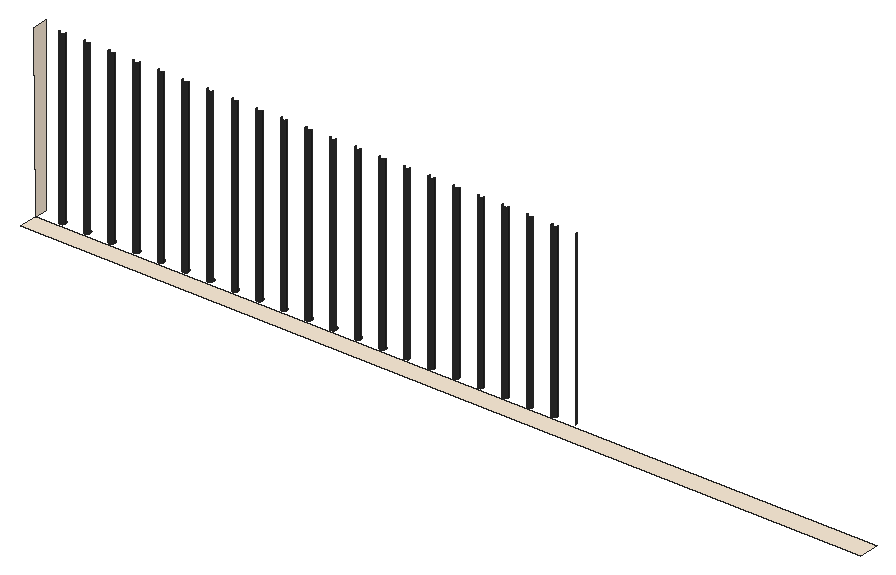
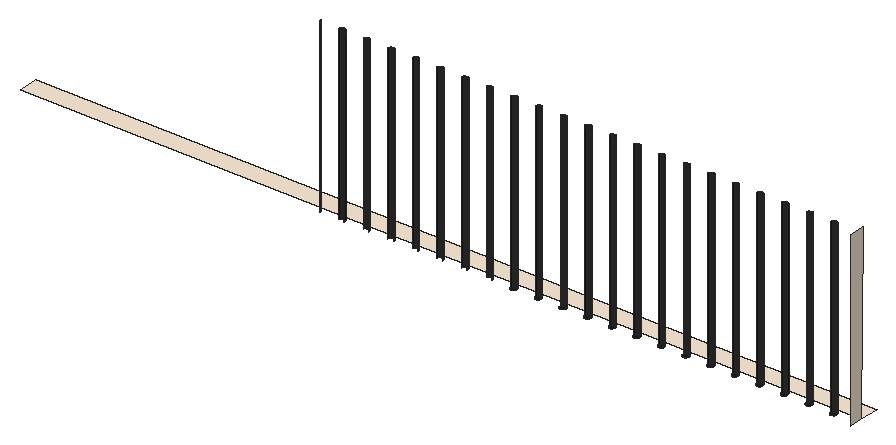
# SketchUp Ruby script. Lengths in inches.
U = 1.inch
M = Sketchup.active_model
def pt(a) = Geom::Point3d.new(a.map { |v| v * U })
def face(e, loops, mat)
  f = e.add_face(loops[0].map { |a| pt(a) })
  loops[1..].each { |l| e.add_face(l.map { |a| pt(a) }).erase! }
  f.material = f.back_material = mat if mat
  f
end
# faces: each face lists its corners as indices into pts; further lists are holes
def faces(e, pts, list, mat = nil) = list.each { |f| face(e, (f[0].is_a?(Array) ? f : [f]).map { |l| l.map { |i| pts[i] } }, mat) }
# xy, xz, yz: faces in a plane at the given z, y or x. An outline is a flat list of corners, or four numbers for a rectangle; further outlines are holes
def ring(l) = l.size == 4 ? [[l[0], l[1]], [l[2], l[1]], [l[2], l[3]], [l[0], l[3]]] : l.each_slice(2).to_a
def flat(e, list, mat, &to3) = list.each { |f| face(e, (f[0].is_a?(Array) ? f : [f]).map { |l| ring(l).map { |u, v| to3.(u, v) } }, mat) }
def xy(e, z, list, mat = nil) = flat(e, list, mat) { |x, y| [x, y, z] }
def xz(e, y, list, mat = nil) = flat(e, list, mat) { |x, z| [x, y, z] }
def yz(e, x, list, mat = nil) = flat(e, list, mat) { |y, z| [x, y, z] }
def lines(e, pts, list) = list.each { |a, b| e.add_line(pt(pts[a]), pt(pts[b])) }
# prism: a flat outline (further loops are holes) pulled along v
def prism(e, loops, v, mat = nil)
  f = face(e, loops, mat); d = Geom::Vector3d.new(v.map { |x| x * U })
  f.pushpull(f.normal.samedirection?(d) ? d.length : -d.length)
end
def box(e, o, s, mat = nil) = prism(e, [[o, [o[0] + s[0], o[1], o[2]], [o[0] + s[0], o[1] + s[1], o[2]], [o[0], o[1] + s[1], o[2]]]], [0, 0, s[2]], mat)
def at(x, y, z, deg = 0) = Geom::Transformation.translation(pt([x, y, z])) * Geom::Transformation.rotation(ORIGIN, Z_AXIS, deg.degrees)
def axes(o, x, y, z) = Geom::Transformation.new([*x, 0, *y, 0, *z, 0, *pt(o).to_a, 1])
def part(name) = M.definitions.add(name)
# library, detail: a bought-in or finely detailed component or shape, given as its bounding box
def library(name, o, s) = part(name).tap { |d| box(d.entities, o, s) }
def detail(e, o, s) = box(e.add_group.entities, o, s)
def put(e, d, t, mat = nil) = e.add_instance(d, t).tap { |i| i.material = mat if mat }
def group(e, t, mat = nil) = e.add_group.tap { |g| g.transformation = t; g.material = mat if mat }.entities
root = M.entities
M.materials.add("[0028_AntiqueWhite]").color = [250, 235, 215]
M.materials.add("[Color M08]").color = [30, 30, 30]
xy(root,177,[[50.75,190.5,206.5625,194.125]],"[0028_AntiqueWhite]")
xy(root,177,[[54.79,194.68,54.65,194.71,54.52,194.79,54.42,194.89,54.35,195.02,54.31,195.16,54.31,195.31,54.34,195.45,54.42,195.58,54.52,195.68,54.65,195.75,54.79,195.79,54.9375,195.79,55.08,195.75,55.21,195.68,55.31,195.58,55.38,195.45,55.42,195.31,55.42,195.16,55.38,195.02,55.3125,194.89,55.21,194.79,55.08,194.72,54.9375,194.68],[59.35,194.68,59.21,194.71,59.09,194.79,58.98,194.89,58.91,195.02,58.87,195.16,58.87,195.31,58.91,195.45,58.98,195.58,59.08,195.68,59.21,195.75,59.35,195.79,59.5,195.79,59.64,195.75,59.77,195.68,59.87,195.58,59.95,195.45,59.98,195.31,59.99,195.16,59.95,195.02,59.875,194.89,59.77,194.79,59.64,194.72,59.5,194.68],[63.92,194.68,63.78,194.71,63.65,194.79,63.54,194.89,63.47,195.02,63.43,195.16,63.43,195.31,63.47,195.45,63.54,195.58,63.65,195.68,63.77,195.75,63.92,195.79,64.0625,195.79,64.2,195.75,64.33,195.68,64.44,195.58,64.51,195.45,64.55,195.31,64.55,195.16,64.51,195.02,64.4375,194.89,64.33,194.79,64.21,194.72,64.0625,194.68],[68.48,194.68,68.34,194.71,68.21,194.79,68.11,194.89,68.03,195.02,67.99,195.16,67.99,195.31,68.03,195.45,68.11,195.58,68.21,195.68,68.34,195.75,68.48,195.79,68.625,195.79,68.77,195.75,68.89,195.68,69,195.58,69.07,195.45,69.11,195.31,69.11,195.16,69.07,195.02,69,194.89,68.9,194.79,68.77,194.72,68.625,194.68],[73.04,194.68,72.9,194.71,72.77,194.79,72.67,194.89,72.6,195.02,72.56,195.16,72.56,195.31,72.59,195.45,72.67,195.58,72.77,195.68,72.9,195.75,73.04,195.79,73.1875,195.79,73.33,195.75,73.46,195.68,73.56,195.58,73.63,195.45,73.67,195.31,73.67,195.16,73.63,195.02,73.5625,194.89,73.46,194.79,73.33,194.72,73.1875,194.68],
  [77.6,194.68,77.46,194.71,77.34,194.79,77.23,194.89,77.16,195.02,77.12,195.16,77.12,195.31,77.16,195.45,77.23,195.58,77.33,195.68,77.46,195.75,77.6,195.79,77.75,195.79,77.89,195.75,78.02,195.68,78.12,195.58,78.2,195.45,78.23,195.31,78.24,195.16,78.2,195.02,78.125,194.89,78.02,194.79,77.89,194.72,77.75,194.68],[82.17,194.68,82.03,194.71,81.9,194.79,81.79,194.89,81.72,195.02,81.68,195.16,81.68,195.31,81.72,195.45,81.79,195.58,81.9,195.68,82.02,195.75,82.17,195.79,82.3125,195.79,82.45,195.75,82.58,195.68,82.69,195.58,82.76,195.45,82.8,195.31,82.8,195.16,82.76,195.02,82.6875,194.89,82.58,194.79,82.46,194.72,82.3125,194.68],[86.73,194.68,86.59,194.71,86.46,194.79,86.36,194.89,86.28,195.02,86.24,195.16,86.24,195.31,86.28,195.45,86.36,195.58,86.46,195.68,86.59,195.75,86.73,195.79,86.875,195.79,87.02,195.75,87.14,195.68,87.25,195.58,87.32,195.45,87.36,195.31,87.36,195.16,87.32,195.02,87.25,194.89,87.15,194.79,87.02,194.72,86.875,194.68],[91.29,194.68,91.15,194.71,91.02,194.79,90.92,194.89,90.85,195.02,90.81,195.16,90.81,195.31,90.84,195.45,90.92,195.58,91.02,195.68,91.15,195.75,91.29,195.79,91.4375,195.79,91.58,195.75,91.71,195.68,91.81,195.58,91.88,195.45,91.92,195.31,91.92,195.16,91.88,195.02,91.8125,194.89,91.71,194.79,91.58,194.72,91.4375,194.68],[95.85,194.68,95.71,194.71,95.59,194.79,95.48,194.89,95.41,195.02,95.37,195.16,95.37,195.31,95.41,195.45,95.48,195.58,95.58,195.68,95.71,195.75,95.85,195.79,96,195.79,96.14,195.75,96.27,195.68,96.37,195.58,96.45,195.45,96.48,195.31,96.49,195.16,96.45,195.02,96.375,194.89,96.27,194.79,96.14,194.72,96,194.68],
  [100.42,194.68,100.28,194.71,100.15,194.79,100.04,194.89,99.97,195.02,99.93,195.16,99.93,195.31,99.97,195.45,100.04,195.58,100.15,195.68,100.27,195.75,100.42,195.79,100.5625,195.79,100.7,195.75,100.83,195.68,100.94,195.58,101.01,195.45,101.05,195.31,101.05,195.16,101.01,195.02,100.9375,194.89,100.83,194.79,100.71,194.72,100.5625,194.68],[104.98,194.68,104.84,194.71,104.71,194.79,104.61,194.89,104.53,195.02,104.49,195.16,104.49,195.31,104.53,195.45,104.61,195.58,104.71,195.68,104.84,195.75,104.98,195.79,105.125,195.79,105.27,195.75,105.39,195.68,105.5,195.58,105.57,195.45,105.61,195.31,105.61,195.16,105.57,195.02,105.5,194.89,105.4,194.79,105.27,194.72,105.125,194.68],[109.54,194.68,109.4,194.71,109.27,194.79,109.17,194.89,109.1,195.02,109.06,195.16,109.06,195.31,109.09,195.45,109.17,195.58,109.27,195.68,109.4,195.75,109.54,195.79,109.6875,195.79,109.83,195.75,109.96,195.68,110.06,195.58,110.13,195.45,110.17,195.31,110.17,195.16,110.13,195.02,110.0625,194.89,109.96,194.79,109.83,194.72,109.6875,194.68],[114.1,194.68,113.96,194.71,113.84,194.79,113.73,194.89,113.66,195.02,113.62,195.16,113.62,195.31,113.66,195.45,113.73,195.58,113.83,195.68,113.96,195.75,114.1,195.79,114.25,195.79,114.39,195.75,114.52,195.68,114.62,195.58,114.7,195.45,114.73,195.31,114.74,195.16,114.7,195.02,114.625,194.89,114.52,194.79,114.39,194.72,114.25,194.68]],"[Color M08]")
xz(root,194.68,[[54.79,177,54.9375,208.66],[59.35,177,59.5,208.66],[63.92,177,64.0625,208.66],[68.48,177,68.625,208.66],[73.04,177,73.1875,208.66],
  [77.6,177,77.75,208.66],[82.17,177,82.3125,208.66],[86.73,177,86.875,208.66],[91.29,177,91.4375,208.66],[95.85,177,96,208.66],
  [100.42,177,100.5625,208.66],[104.98,177,105.125,208.66],[109.54,177,109.6875,208.66],[114.1,177,114.25,208.66],[118.67,177,118.8125,208.66],
  [123.23,177,123.375,208.66],[127.79,177,127.9375,208.66],[132.35,177,132.5,208.66],[136.92,177,137.0625,208.66],[141.48,177,141.625,208.66],
  [146.04,177,146.1875,208.66]],"[Color M08]")
yz(root,50.75,[[194.125,177,196.4375,177,196.4375,208.66,193.58,208.66]],"[0028_AntiqueWhite]")
yz(root,54.31,[[195.16,177,195.31,208.66]],"[Color M08]")
yz(root,58.87,[[195.16,177,195.31,208.66]],"[Color M08]")
yz(root,63.43,[[195.16,177,195.31,208.66]],"[Color M08]")
yz(root,67.99,[[195.16,177,195.31,208.66]],"[Color M08]")
yz(root,72.56,[[195.16,177,195.31,208.66]],"[Color M08]")
yz(root,77.12,[[195.16,177,195.31,208.66]],"[Color M08]")
yz(root,81.68,[[195.16,177,195.31,208.66]],"[Color M08]")
yz(root,86.24,[[195.16,177,195.31,208.66]],"[Color M08]")
yz(root,90.81,[[195.16,177,195.31,208.66]],"[Color M08]")
yz(root,95.37,[[195.16,177,195.31,208.66]],"[Color M08]")
yz(root,99.93,[[195.16,177,195.31,208.66]],"[Color M08]")
yz(root,104.49,[[195.16,177,195.31,208.66]],"[Color M08]")
yz(root,109.06,[[195.16,177,195.31,208.66]],"[Color M08]")
yz(root,113.62,[[195.16,177,195.31,208.66]],"[Color M08]")
yz(root,118.18,[[195.16,177,195.31,208.66]],"[Color M08]")
yz(root,122.74,[[195.16,177,195.31,208.66]],"[Color M08]")
yz(root,127.31,[[195.16,177,195.31,208.66]],"[Color M08]")
yz(root,131.87,[[195.16,177,195.31,208.66]],"[Color M08]")
yz(root,136.43,[[195.16,177,195.31,208.66]],"[Color M08]")
yz(root,140.99,[[195.16,177,195.31,208.66]],"[Color M08]")
yz(root,145.56,[[195.16,177,195.31,208.66]],"[Color M08]")
yz(root,150.12,[[195.16,177,195.31,208.66]],"[Color M08]")
p = [[54.52,194.79,177],[54.65,194.71,177],[54.65,194.71,208.66],[54.52,194.79,208.66],[54.79,194.68,177],[54.79,194.68,208.66],
  [54.9375,194.68,177],[55.08,194.72,177],[55.08,194.72,208.66],[54.9375,194.68,208.66],[55.21,194.79,177],[55.21,194.79,208.66],
  [59.09,194.79,177],[59.21,194.71,177],[59.21,194.71,208.66],[59.09,194.79,208.66],[59.35,194.68,177],[59.35,194.68,208.66],
  [59.5,194.68,177],[59.64,194.72,177],[59.64,194.72,208.66],[59.5,194.68,208.66],[59.77,194.79,177],[59.77,194.79,208.66],
  [63.65,194.79,177],[63.78,194.71,177],[63.78,194.71,208.66],[63.65,194.79,208.66],[63.92,194.68,177],[63.92,194.68,208.66],
  [64.0625,194.68,177],[64.21,194.72,177],[64.21,194.72,208.66],[64.0625,194.68,208.66],[64.33,194.79,177],[64.33,194.79,208.66],
  [68.21,194.79,177],[68.34,194.71,177],[68.34,194.71,208.66],[68.21,194.79,208.66],[68.48,194.68,177],[68.48,194.68,208.66],
  [68.625,194.68,177],[68.77,194.72,177],[68.77,194.72,208.66],[68.625,194.68,208.66],[68.9,194.79,177],[68.9,194.79,208.66],
  [72.77,194.79,177],[72.9,194.71,177],[72.9,194.71,208.66],[72.77,194.79,208.66],[73.04,194.68,177],[73.04,194.68,208.66],
  [73.1875,194.68,177],[73.33,194.72,177],[73.33,194.72,208.66],[73.1875,194.68,208.66],[73.46,194.79,177],[73.46,194.79,208.66],
  [77.34,194.79,177],[77.46,194.71,177],[77.46,194.71,208.66],[77.34,194.79,208.66],[77.6,194.68,177],[77.6,194.68,208.66],
  [77.75,194.68,177],[77.89,194.72,177],[77.89,194.72,208.66],[77.75,194.68,208.66],[78.02,194.79,177],[78.02,194.79,208.66],
  [81.9,194.79,177],[82.03,194.71,177],[82.03,194.71,208.66],[81.9,194.79,208.66],[82.17,194.68,177],[82.17,194.68,208.66],
  [82.3125,194.68,177],[82.46,194.72,177],[82.46,194.72,208.66],[82.3125,194.68,208.66],[82.58,194.79,177],[82.58,194.79,208.66],
  [86.46,194.79,177],[86.59,194.71,177],[86.59,194.71,208.66],[86.46,194.79,208.66],[86.73,194.68,177],[86.73,194.68,208.66],
  [86.875,194.68,177],[87.02,194.72,177],[87.02,194.72,208.66],[86.875,194.68,208.66],[87.15,194.79,177],[87.15,194.79,208.66],
  [91.02,194.79,177],[91.15,194.71,177],[91.15,194.71,208.66],[91.02,194.79,208.66],[91.29,194.68,177],[91.29,194.68,208.66],
  [91.4375,194.68,177],[91.58,194.72,177],[91.58,194.72,208.66],[91.4375,194.68,208.66],[91.71,194.79,177],[91.71,194.79,208.66],
  [95.59,194.79,177],[95.71,194.71,177],[95.71,194.71,208.66],[95.59,194.79,208.66],[95.85,194.68,177],[95.85,194.68,208.66],
  [96,194.68,177],[96.14,194.72,177],[96.14,194.72,208.66],[96,194.68,208.66],[96.27,194.79,177],[96.27,194.79,208.66],
  [100.15,194.79,177],[100.28,194.71,177],[100.28,194.71,208.66],[100.15,194.79,208.66],[100.42,194.68,177],[100.42,194.68,208.66],
  [100.5625,194.68,177],[100.71,194.72,177],[100.71,194.72,208.66],[100.5625,194.68,208.66],[100.83,194.79,177],[100.83,194.79,208.66],
  [104.71,194.79,177],[104.84,194.71,177],[104.84,194.71,208.66],[104.71,194.79,208.66],[104.98,194.68,177],[104.98,194.68,208.66],
  [105.125,194.68,177],[105.27,194.72,177],[105.27,194.72,208.66],[105.125,194.68,208.66],[105.4,194.79,177],[105.4,194.79,208.66],
  [109.27,194.79,177],[109.4,194.71,177],[109.4,194.71,208.66],[109.27,194.79,208.66],[109.54,194.68,177],[109.54,194.68,208.66],
  [109.6875,194.68,177],[109.83,194.72,177],[109.83,194.72,208.66],[109.6875,194.68,208.66],[109.96,194.79,177],[109.96,194.79,208.66],
  [113.84,194.79,177],[113.96,194.71,177],[113.96,194.71,208.66],[113.84,194.79,208.66],[114.1,194.68,177],[114.1,194.68,208.66],
  [114.25,194.68,177],[114.39,194.72,177],[114.39,194.72,208.66],[114.25,194.68,208.66],[114.52,194.79,177],[114.52,194.79,208.66],
  [118.4,194.79,177],[118.53,194.71,177],[118.53,194.71,208.66],[118.4,194.79,208.66],[118.67,194.68,177],[118.67,194.68,208.66],
  [118.8125,194.68,177],[118.96,194.72,177],[118.96,194.72,208.66],[118.8125,194.68,208.66],[119.08,194.79,177],[119.08,194.79,208.66],
  [122.96,194.79,177],[123.09,194.71,177],[123.09,194.71,208.66],[122.96,194.79,208.66],[123.23,194.68,177],[123.23,194.68,208.66],
  [123.375,194.68,177],[123.52,194.72,177],[123.52,194.72,208.66],[123.375,194.68,208.66],[123.65,194.79,177],[123.65,194.79,208.66],
  [127.52,194.79,177],[127.65,194.71,177],[127.65,194.71,208.66],[127.52,194.79,208.66],[127.79,194.68,177],[127.79,194.68,208.66],
  [127.9375,194.68,177],[128.08,194.72,177],[128.08,194.72,208.66],[127.9375,194.68,208.66],[128.21,194.79,177],[128.21,194.79,208.66],
  [132.09,194.79,177],[132.21,194.71,177],[132.21,194.71,208.66],[132.09,194.79,208.66],[132.35,194.68,177],[132.35,194.68,208.66],
  [132.5,194.68,177],[132.64,194.72,177],[132.64,194.72,208.66],[132.5,194.68,208.66],[132.77,194.79,177],[132.77,194.79,208.66],
  [136.65,194.79,177],[136.78,194.71,177],[136.78,194.71,208.66],[136.65,194.79,208.66],[136.92,194.68,177],[136.92,194.68,208.66],
  [137.0625,194.68,177],[137.21,194.72,177],[137.21,194.72,208.66],[137.0625,194.68,208.66],[137.33,194.79,177],[137.33,194.79,208.66],
  [141.21,194.79,177],[141.34,194.71,177],[141.34,194.71,208.66],[141.21,194.79,208.66],[141.48,194.68,177],[141.48,194.68,208.66],
  [141.625,194.68,177],[141.77,194.72,177],[141.77,194.72,208.66],[141.625,194.68,208.66],[141.9,194.79,177],[141.9,194.79,208.66],
  [145.77,194.79,177],[145.9,194.71,177],[145.9,194.71,208.66],[145.77,194.79,208.66],[146.04,194.68,177],[146.04,194.68,208.66],
  [146.1875,194.68,177],[146.33,194.72,177],[146.33,194.72,208.66],[146.1875,194.68,208.66],[146.46,194.79,177],[146.46,194.79,208.66],
  [54.42,194.89,177],[54.42,194.89,208.66],[55.3125,194.89,177],[55.3125,194.89,208.66],[58.98,194.89,177],[58.98,194.89,208.66],
  [59.875,194.89,177],[59.875,194.89,208.66],[63.54,194.89,177],[63.54,194.89,208.66],[64.4375,194.89,177],[64.4375,194.89,208.66],
  [68.11,194.89,177],[68.11,194.89,208.66],[69,194.89,177],[69,194.89,208.66],[72.67,194.89,177],[72.67,194.89,208.66],
  [73.5625,194.89,177],[73.5625,194.89,208.66],[77.23,194.89,177],[77.23,194.89,208.66],[78.125,194.89,177],[78.125,194.89,208.66],
  [81.79,194.89,177],[81.79,194.89,208.66],[82.6875,194.89,177],[82.6875,194.89,208.66],[86.36,194.89,177],[86.36,194.89,208.66],
  [87.25,194.89,177],[87.25,194.89,208.66],[90.92,194.89,177],[90.92,194.89,208.66],[91.8125,194.89,177],[91.8125,194.89,208.66],
  [95.48,194.89,177],[95.48,194.89,208.66],[96.375,194.89,177],[96.375,194.89,208.66],[100.04,194.89,177],[100.04,194.89,208.66],
  [100.9375,194.89,177],[100.9375,194.89,208.66],[104.61,194.89,177],[104.61,194.89,208.66],[105.5,194.89,177],[105.5,194.89,208.66],
  [109.17,194.89,177],[109.17,194.89,208.66],[110.0625,194.89,177],[110.0625,194.89,208.66],[113.73,194.89,177],[113.73,194.89,208.66],
  [114.625,194.89,177],[114.625,194.89,208.66],[118.29,194.89,177],[118.29,194.89,208.66],[119.1875,194.89,177],[119.1875,194.89,208.66],
  [122.86,194.89,177],[122.86,194.89,208.66],[123.75,194.89,177],[123.75,194.89,208.66],[127.42,194.89,177],[127.42,194.89,208.66],
  [128.3125,194.89,177],[128.3125,194.89,208.66],[131.98,194.89,177],[131.98,194.89,208.66],[132.875,194.89,177],[132.875,194.89,208.66],
  [136.54,194.89,177],[136.54,194.89,208.66],[137.4375,194.89,177],[137.4375,194.89,208.66],[141.11,194.89,177],[141.11,194.89,208.66],
  [142,194.89,177],[142,194.89,208.66],[145.67,194.89,177],[145.67,194.89,208.66],[146.5625,194.89,177],[146.5625,194.89,208.66],
  [54.35,195.02,177],[54.35,195.02,208.66],[55.38,195.02,177],[55.38,195.02,208.66],[58.91,195.02,177],[58.91,195.02,208.66],
  [59.95,195.02,177],[59.95,195.02,208.66],[63.47,195.02,177],[63.47,195.02,208.66],[64.51,195.02,177],[64.51,195.02,208.66],
  [68.03,195.02,177],[68.03,195.02,208.66],[69.07,195.02,177],[69.07,195.02,208.66],[72.6,195.02,177],[72.6,195.02,208.66],
  [73.63,195.02,177],[73.63,195.02,208.66],[77.16,195.02,177],[77.16,195.02,208.66],[78.2,195.02,177],[78.2,195.02,208.66],
  [81.72,195.02,177],[81.72,195.02,208.66],[82.76,195.02,177],[82.76,195.02,208.66],[86.28,195.02,177],[86.28,195.02,208.66],
  [87.32,195.02,177],[87.32,195.02,208.66],[90.85,195.02,177],[90.85,195.02,208.66],[91.88,195.02,177],[91.88,195.02,208.66],
  [95.41,195.02,177],[95.41,195.02,208.66],[96.45,195.02,177],[96.45,195.02,208.66],[99.97,195.02,177],[99.97,195.02,208.66],
  [101.01,195.02,177],[101.01,195.02,208.66],[104.53,195.02,177],[104.53,195.02,208.66],[105.57,195.02,177],[105.57,195.02,208.66],
  [109.1,195.02,177],[109.1,195.02,208.66],[110.13,195.02,177],[110.13,195.02,208.66],[113.66,195.02,177],[113.66,195.02,208.66],
  [114.7,195.02,177],[114.7,195.02,208.66],[118.22,195.02,177],[118.22,195.02,208.66],[119.26,195.02,177],[119.26,195.02,208.66],
  [122.78,195.02,177],[122.78,195.02,208.66],[123.82,195.02,177],[123.82,195.02,208.66],[127.35,195.02,177],[127.35,195.02,208.66],
  [128.38,195.02,177],[128.38,195.02,208.66],[131.91,195.02,177],[131.91,195.02,208.66],[132.95,195.02,177],[132.95,195.02,208.66],
  [136.47,195.02,177],[136.47,195.02,208.66],[137.51,195.02,177],[137.51,195.02,208.66],[141.03,195.02,177],[141.03,195.02,208.66],
  [142.07,195.02,177],[142.07,195.02,208.66],[145.6,195.02,177],[145.6,195.02,208.66],[146.63,195.02,177],[146.63,195.02,208.66],
  [150.16,195.02,177],[150.23,194.89,177],[150.23,194.89,208.66],[150.16,195.02,208.66],[54.31,195.16,177],[54.31,195.16,208.66],
  [55.42,195.16,177],[55.42,195.16,208.66],[58.87,195.16,177],[58.87,195.16,208.66],[59.99,195.16,177],[59.99,195.16,208.66],
  [63.43,195.16,177],[63.43,195.16,208.66],[64.55,195.16,177],[64.55,195.16,208.66],[67.99,195.16,177],[67.99,195.16,208.66],
  [69.11,195.16,177],[69.11,195.16,208.66],[72.56,195.16,177],[72.56,195.16,208.66],[73.67,195.16,177],[73.67,195.16,208.66],
  [77.12,195.16,177],[77.12,195.16,208.66],[78.24,195.16,177],[78.24,195.16,208.66],[81.68,195.16,177],[81.68,195.16,208.66],
  [82.8,195.16,177],[82.8,195.16,208.66],[86.24,195.16,177],[86.24,195.16,208.66],[87.36,195.16,177],[87.36,195.16,208.66],
  [90.81,195.16,177],[90.81,195.16,208.66],[91.92,195.16,177],[91.92,195.16,208.66],[95.37,195.16,177],[95.37,195.16,208.66],
  [96.49,195.16,177],[96.49,195.16,208.66],[99.93,195.16,177],[99.93,195.16,208.66],[101.05,195.16,177],[101.05,195.16,208.66],
  [104.49,195.16,177],[104.49,195.16,208.66],[105.61,195.16,177],[105.61,195.16,208.66],[109.06,195.16,177],[109.06,195.16,208.66],
  [110.17,195.16,177],[110.17,195.16,208.66],[113.62,195.16,177],[113.62,195.16,208.66],[114.74,195.16,177],[114.74,195.16,208.66],
  [118.18,195.16,177],[118.18,195.16,208.66],[119.3,195.16,177],[119.3,195.16,208.66],[122.74,195.16,177],[122.74,195.16,208.66],
  [123.86,195.16,177],[123.86,195.16,208.66],[127.31,195.16,177],[127.31,195.16,208.66],[128.42,195.16,177],[128.42,195.16,208.66],
  [131.87,195.16,177],[131.87,195.16,208.66],[132.99,195.16,177],[132.99,195.16,208.66],[136.43,195.16,177],[136.43,195.16,208.66],
  [137.55,195.16,177],[137.55,195.16,208.66],[140.99,195.16,177],[140.99,195.16,208.66],[142.11,195.16,177],[142.11,195.16,208.66],
  [145.56,195.16,177],[145.56,195.16,208.66],[146.67,195.16,177],[146.67,195.16,208.66],[150.12,195.16,177],[150.12,195.16,208.66]]
faces(root,p,[[0,1,2,3],[1,4,5,2],[6,7,8,9],[7,10,11,8],[12,13,14,15],[13,16,17,14],[18,19,20,21],[19,22,23,20],
  [24,25,26,27],[25,28,29,26],[30,31,32,33],[31,34,35,32],[36,37,38,39],[37,40,41,38],[42,43,44,45],[43,46,47,44],
  [48,49,50,51],[49,52,53,50],[54,55,56,57],[55,58,59,56],[60,61,62,63],[61,64,65,62],[66,67,68,69],[67,70,71,68],
  [72,73,74,75],[73,76,77,74],[78,79,80,81],[79,82,83,80],[84,85,86,87],[85,88,89,86],[90,91,92,93],[91,94,95,92],
  [96,97,98,99],[97,100,101,98],[102,103,104,105],[103,106,107,104],[108,109,110,111],[109,112,113,110],[114,115,116,117],[115,118,119,116],
  [120,121,122,123],[121,124,125,122],[126,127,128,129],[127,130,131,128],[132,133,134,135],[133,136,137,134],[138,139,140,141],[139,142,143,140],
  [144,145,146,147],[145,148,149,146],[150,151,152,153],[151,154,155,152],[156,157,158,159],[157,160,161,158],[162,163,164,165],[163,166,167,164],
  [168,169,170,171],[169,172,173,170],[174,175,176,177],[175,178,179,176],[180,181,182,183],[181,184,185,182],[186,187,188,189],[187,190,191,188],
  [192,193,194,195],[193,196,197,194],[198,199,200,201],[199,202,203,200],[204,205,206,207],[205,208,209,206],[210,211,212,213],[211,214,215,212],
  [216,217,218,219],[217,220,221,218],[222,223,224,225],[223,226,227,224],[228,229,230,231],[229,232,233,230],[234,235,236,237],[235,238,239,236],
  [240,241,242,243],[241,244,245,242],[246,247,248,249],[247,250,251,248],[252,0,3,253],[10,254,255,11],[256,12,15,257],[22,258,259,23],
  [260,24,27,261],[34,262,263,35],[264,36,39,265],[46,266,267,47],[268,48,51,269],[58,270,271,59],[272,60,63,273],[70,274,275,71],
  [276,72,75,277],[82,278,279,83],[280,84,87,281],[94,282,283,95],[284,96,99,285],[106,286,287,107],[288,108,111,289],[118,290,291,119],
  [292,120,123,293],[130,294,295,131],[296,132,135,297],[142,298,299,143],[300,144,147,301],[154,302,303,155],[304,156,159,305],[166,306,307,167],
  [308,168,171,309],[178,310,311,179],[312,180,183,313],[190,314,315,191],[316,192,195,317],[202,318,319,203],[320,204,207,321],[214,322,323,215],
  [324,216,219,325],[226,326,327,227],[328,228,231,329],[238,330,331,239],[332,240,243,333],[250,334,335,251],[336,252,253,337],[254,338,339,255],
  [340,256,257,341],[258,342,343,259],[344,260,261,345],[262,346,347,263],[348,264,265,349],[266,350,351,267],[352,268,269,353],[270,354,355,271],
  [356,272,273,357],[274,358,359,275],[360,276,277,361],[278,362,363,279],[364,280,281,365],[282,366,367,283],[368,284,285,369],[286,370,371,287],
  [372,288,289,373],[290,374,375,291],[376,292,293,377],[294,378,379,295],[380,296,297,381],[298,382,383,299],[384,300,301,385],[302,386,387,303],
  [388,304,305,389],[306,390,391,307],[392,308,309,393],[310,394,395,311],[396,312,313,397],[314,398,399,315],[400,316,317,401],[318,402,403,319],
  [404,320,321,405],[322,406,407,323],[408,324,325,409],[326,410,411,327],[412,328,329,413],[330,414,415,331],[416,332,333,417],[334,418,419,335],
  [420,421,422,423],[424,336,337,425],[338,426,427,339],[428,340,341,429],[342,430,431,343],[432,344,345,433],[346,434,435,347],[436,348,349,437],
  [350,438,439,351],[440,352,353,441],[354,442,443,355],[444,356,357,445],[358,446,447,359],[448,360,361,449],[362,450,451,363],[452,364,365,453],
  [366,454,455,367],[456,368,369,457],[370,458,459,371],[460,372,373,461],[374,462,463,375],[464,376,377,465],[378,466,467,379],[468,380,381,469],
  [382,470,471,383],[472,384,385,473],[386,474,475,387],[476,388,389,477],[390,478,479,391],[480,392,393,481],[394,482,483,395],[484,396,397,485],
  [398,486,487,399],[488,400,401,489],[402,490,491,403],[492,404,405,493],[406,494,495,407],[496,408,409,497],[410,498,499,411],[500,412,413,501],
  [414,502,503,415],[504,416,417,505],[418,506,507,419],[508,420,423,509]],"[Color M08]")
